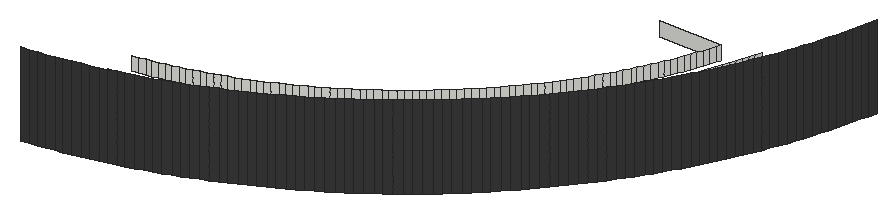
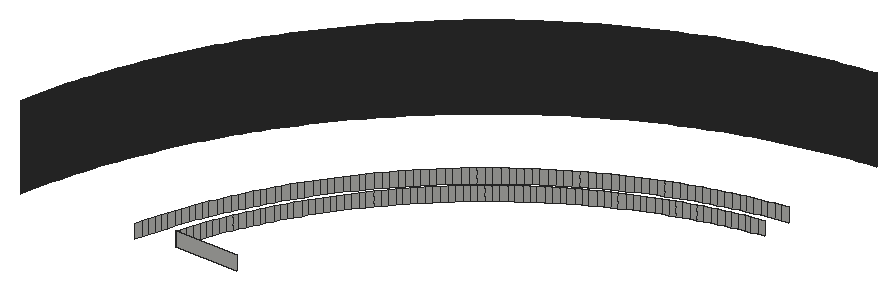
# SketchUp Ruby script. Lengths in inches.
U = 1.inch
M = Sketchup.active_model
def pt(a) = Geom::Point3d.new(a.map { |v| v * U })
def face(e, loops, mat)
  f = e.add_face(loops[0].map { |a| pt(a) })
  loops[1..].each { |l| e.add_face(l.map { |a| pt(a) }).erase! }
  f.material = f.back_material = mat if mat
  f
end
# faces: each face lists its corners as indices into pts; further lists are holes
def faces(e, pts, list, mat = nil) = list.each { |f| face(e, (f[0].is_a?(Array) ? f : [f]).map { |l| l.map { |i| pts[i] } }, mat) }
# xy, xz, yz: faces in a plane at the given z, y or x. An outline is a flat list of corners, or four numbers for a rectangle; further outlines are holes
def ring(l) = l.size == 4 ? [[l[0], l[1]], [l[2], l[1]], [l[2], l[3]], [l[0], l[3]]] : l.each_slice(2).to_a
def flat(e, list, mat, &to3) = list.each { |f| face(e, (f[0].is_a?(Array) ? f : [f]).map { |l| ring(l).map { |u, v| to3.(u, v) } }, mat) }
def xy(e, z, list, mat = nil) = flat(e, list, mat) { |x, y| [x, y, z] }
def xz(e, y, list, mat = nil) = flat(e, list, mat) { |x, z| [x, y, z] }
def yz(e, x, list, mat = nil) = flat(e, list, mat) { |y, z| [x, y, z] }
def lines(e, pts, list) = list.each { |a, b| e.add_line(pt(pts[a]), pt(pts[b])) }
# prism: a flat outline (further loops are holes) pulled along v
def prism(e, loops, v, mat = nil)
  f = face(e, loops, mat); d = Geom::Vector3d.new(v.map { |x| x * U })
  f.pushpull(f.normal.samedirection?(d) ? d.length : -d.length)
end
def box(e, o, s, mat = nil) = prism(e, [[o, [o[0] + s[0], o[1], o[2]], [o[0] + s[0], o[1] + s[1], o[2]], [o[0], o[1] + s[1], o[2]]]], [0, 0, s[2]], mat)
def at(x, y, z, deg = 0) = Geom::Transformation.translation(pt([x, y, z])) * Geom::Transformation.rotation(ORIGIN, Z_AXIS, deg.degrees)
def axes(o, x, y, z) = Geom::Transformation.new([*x, 0, *y, 0, *z, 0, *pt(o).to_a, 1])
def part(name) = M.definitions.add(name)
# library, detail: a bought-in or finely detailed component or shape, given as its bounding box
def library(name, o, s) = part(name).tap { |d| box(d.entities, o, s) }
def detail(e, o, s) = box(e.add_group.entities, o, s)
def put(e, d, t, mat = nil) = e.add_instance(d, t).tap { |i| i.material = mat if mat }
def group(e, t, mat = nil) = e.add_group.tap { |g| g.transformation = t; g.material = mat if mat }.entities
root = M.entities
M.materials.add("1496 AP 8293 CARBON COPY").color = [58, 58, 58]
xz(root,80,[[198,258,200.2,258.5]])
p = [[188.01,64.22,261],[187.74,64.18,261],[187.74,64.18,258],[188.01,64.22,258],[188.29,64.26,261],[188.29,64.26,258],
  [188.56,64.3,261],[188.56,64.3,258],[188.83,64.35,261],[188.83,64.35,258],[189.1,64.4,261],[189.1,64.4,258],
  [189.37,64.46,261],[189.37,64.46,258],[189.63,64.52,261],[189.63,64.52,258],[189.9,64.58,261],[189.9,64.58,258],
  [190.17,64.65,261],[190.17,64.65,258],[190.44,64.72,261],[190.44,64.72,258],[190.7,64.79,261],[190.7,64.79,258],
  [190.96,64.86,261],[190.96,64.86,258],[191.23,64.94,261],[191.23,64.94,258],[191.49,65.03,261],[191.49,65.03,258],
  [191.75,65.11,261],[191.75,65.11,258],[192.01,65.2,261],[192.01,65.2,258],[192.27,65.3,261],[192.27,65.3,258],
  [192.53,65.39,261],[192.53,65.39,258],[192.78,65.49,261],[192.78,65.49,258],[193.04,65.6,261],[193.04,65.6,258],
  [193.29,65.71,261],[193.29,65.71,258],[193.54,65.82,261],[193.54,65.82,258],[193.79,65.93,261],[193.79,65.93,258],
  [194.04,66.05,261],[194.04,66.05,258],[194.29,66.17,261],[194.29,66.17,258],[194.53,66.29,261],[194.53,66.29,258],
  [194.78,66.42,261],[194.78,66.42,258],[195.02,66.54,261],[195.02,66.54,258],[195.26,66.68,261],[195.26,66.68,258],
  [195.5,66.8125,261],[195.5,66.8125,258],[195.74,66.95,261],[195.74,66.95,258],[195.97,67.09,261],[195.97,67.09,258],
  [196.21,67.24,261],[196.21,67.24,258],[196.4375,67.39,261],[196.4375,67.39,258],[196.67,67.54,261],[196.67,67.54,258],
  [196.89,67.69,261],[196.89,67.69,258],[197.12,67.85,261],[197.12,67.85,258],[197.34,68.01,261],[197.34,68.01,258],
  [197.56,68.17,261],[197.56,68.17,258],[187.88,68.25,258],[187.66,68.21,258],[187.66,68.21,258.5],[187.88,68.25,258.5],
  [188.1,68.28,258],[188.1,68.28,258.5],[197.78,68.34,261],[197.78,68.34,258],[188.32,68.33,258],[188.32,68.33,258.5],
  [188.53,68.37,258],[188.53,68.37,258.5],[198,68.51,261],[198,68.51,258],[188.75,68.42,258],[188.75,68.42,258.5],
  [188.97,68.47,258],[188.97,68.47,258.5],[189.18,68.52,258],[189.18,68.52,258.5],[189.4,68.58,258],[189.4,68.58,258.5],
  [198.22,68.68,261],[198.22,68.68,258],[189.61,68.64,258],[189.61,68.64,258.5],[189.83,68.7,258],[189.83,68.7,258.5],
  [190.04,68.76,258],[190.04,68.76,258.5],[198.43,68.85,261],[198.43,68.85,258],[190.25,68.83,258],[190.25,68.83,258.5],
  [190.46,68.9,258],[190.46,68.9,258.5],[190.67,68.98,258],[190.67,68.98,258.5],[198.64,69.03,261],[198.64,69.03,258],
  [190.88,69.05,258],[190.88,69.05,258.5],[198.85,69.21,261],[198.85,69.21,258],[191.09,69.13,258],[191.09,69.13,258.5],
  [191.3,69.21,258],[191.3,69.21,258.5],[187.71,69.23,258],[187.92,69.27,258],[187.92,69.27,258.5],[187.71,69.23,258.5],
  [191.51,69.29,258],[191.51,69.29,258.5],[199.05,69.39,261],[199.05,69.39,258],[188.12,69.31,258],[188.12,69.31,258.5],
  [188.33,69.35,258],[188.33,69.35,258.5],[188.53,69.39,258],[188.53,69.39,258.5],[191.71,69.38,258],[191.71,69.38,258.5],
  [188.74,69.44,258],[188.74,69.44,258.5],[188.9375,69.49,258],[188.9375,69.49,258.5],[191.91,69.47,258],[191.91,69.47,258.5],
  [199.25,69.58,261],[199.25,69.58,258],[189.14,69.55,258],[189.14,69.55,258.5],[189.34,69.6,258],[189.34,69.6,258.5],
  [192.12,69.5625,258],[192.12,69.5625,258.5],[189.54,69.66,258],[189.54,69.66,258.5],[192.32,69.66,258],[192.32,69.66,258.5],
  [199.46,69.77,261],[199.46,69.77,258],[189.74,69.72,258],[189.74,69.72,258.5],[189.94,69.78,258],[189.94,69.78,258.5],
  [192.52,69.75,258],[192.52,69.75,258.5],[190.14,69.85,258],[190.14,69.85,258.5],[190.34,69.92,258],[190.34,69.92,258.5],
  [192.72,69.85,258],[192.72,69.85,258.5],[199.65,69.96,261],[199.65,69.96,258],[190.54,69.99,258],[190.54,69.99,258.5],
  [192.92,69.96,258],[192.92,69.96,258.5],[190.73,70.0625,258],[190.73,70.0625,258.5],[193.11,70.06,258],[193.11,70.06,258.5],
  [199.85,70.15,261],[199.85,70.15,258],[190.93,70.14,258],[190.93,70.14,258.5],[191.12,70.22,258],[191.12,70.22,258.5],
  [193.31,70.17,258],[193.31,70.17,258.5],[191.32,70.3,258],[191.32,70.3,258.5],[193.5,70.28,258],[193.5,70.28,258.5],
  [200.04,70.35,261],[200.04,70.35,258],[191.51,70.38,258],[191.51,70.38,258.5],[193.69,70.39,258],[193.69,70.39,258.5],
  [200.23,70.54,261],[200.23,70.54,258],[191.7,70.47,258],[191.7,70.47,258.5],[193.88,70.51,258],[193.88,70.51,258.5],
  [191.89,70.56,258],[191.89,70.56,258.5],[194.07,70.62,258],[194.07,70.62,258.5],[200.42,70.75,261],[200.42,70.75,258],
  [192.08,70.65,258],[192.08,70.65,258.5],[194.26,70.74,258],[194.26,70.74,258.5],[192.26,70.74,258],[192.26,70.74,258.5],
  [192.45,70.84,258],[192.45,70.84,258.5],[194.44,70.87,258],[194.44,70.87,258.5],[200.61,70.95,261],[200.61,70.95,258],
  [192.63,70.9375,258],[192.63,70.9375,258.5],[192.82,71.04,258],[192.82,71.04,258.5],[194.63,70.99,258],[194.63,70.99,258.5],
  [200.79,71.15,261],[200.79,71.15,258],[193,71.14,258],[193,71.14,258.5],[194.8125,71.12,258],[194.8125,71.12,258.5],
  [193.18,71.25,258],[193.18,71.25,258.5],[194.99,71.25,258],[194.99,71.25,258.5],[193.36,71.36,258],[193.36,71.36,258.5],
  [195.17,71.38,258],[195.17,71.38,258.5],[200.97,71.36,261],[200.97,71.36,258],[193.54,71.47,258],[193.54,71.47,258.5],
  [195.35,71.51,258],[195.35,71.51,258.5],[201.15,71.57,261],[201.15,71.57,258],[193.71,71.58,258],[193.71,71.58,258.5],
  [195.52,71.65,258],[195.52,71.65,258.5],[193.89,71.7,258],[193.89,71.7,258.5],[195.7,71.79,258],[195.7,71.79,258.5],
  [201.32,71.78,261],[201.32,71.78,258],[194.0625,71.8125,258],[194.0625,71.8125,258.5],[194.23,71.93,258],[194.23,71.93,258.5],
  [195.87,71.93,258],[195.87,71.93,258.5],[201.49,72,261],[201.49,72,258],[194.4,72.06,258],[194.4,72.06,258.5],
  [196.04,72.07,258],[196.04,72.07,258.5],[201.66,72.22,261],[201.66,72.22,258],[194.57,72.18,258],[194.57,72.18,258.5],
  [196.21,72.22,258],[196.21,72.22,258.5],[194.74,72.31,258],[194.74,72.31,258.5],[196.375,72.37,258],[196.375,72.37,258.5],
  [201.83,72.44,261],[201.83,72.44,258],[194.91,72.44,258],[194.91,72.44,258.5],[195.07,72.57,258],[195.07,72.57,258.5],
  [196.54,72.52,258],[196.54,72.52,258.5],[201.99,72.66,261],[201.99,72.66,258],[196.7,72.67,258],[196.7,72.67,258.5],
  [195.23,72.7,258],[195.23,72.7,258.5],[195.39,72.83,258],[195.39,72.83,258.5],[196.86,72.82,258],[196.86,72.82,258.5],
  [202.15,72.88,261],[202.15,72.88,258],[195.55,72.97,258],[195.55,72.97,258.5],[197.02,72.98,258],[197.02,72.98,258.5],
  [202.31,73.11,261],[202.31,73.11,258],[195.71,73.11,258],[195.71,73.11,258.5],[197.18,73.14,258],[197.18,73.14,258.5],
  [195.86,73.25,258],[195.86,73.25,258.5],[197.33,73.3,258],[197.33,73.3,258.5],[202.46,73.33,261],[202.46,73.33,258],
  [196.01,73.39,258],[196.01,73.39,258.5],[197.48,73.46,258],[197.48,73.46,258.5],[202.61,73.5625,261],[202.61,73.5625,258],
  [196.16,73.54,258],[196.16,73.54,258.5],[196.3125,73.6875,258],[196.3125,73.6875,258.5],[197.63,73.625,258],[197.63,73.625,258.5],
  [197.78,73.79,258],[197.78,73.79,258.5],[202.76,73.79,261],[202.76,73.79,258],[196.46,73.84,258],[196.46,73.84,258.5],
  [196.61,73.99,258],[196.61,73.99,258.5],[197.93,73.96,258],[197.93,73.96,258.5],[202.91,74.03,261],[202.91,74.03,258],
  [196.75,74.14,258],[196.75,74.14,258.5],[198.07,74.13,258],[198.07,74.13,258.5],[203.05,74.26,261],[203.05,74.26,258],
  [196.89,74.29,258],[196.89,74.29,258.5],[198.21,74.3,258],[198.21,74.3,258.5],[197.03,74.45,258],[197.03,74.45,258.5],
  [198.35,74.48,258],[198.35,74.48,258.5],[203.1875,74.5,261],[203.1875,74.5,258],[197.17,74.61,258],[197.17,74.61,258.5],
  [198.49,74.65,258],[198.49,74.65,258.5],[203.32,74.74,261],[203.32,74.74,258],[197.3,74.77,258],[197.3,74.77,258.5],
  [198.62,74.83,258],[198.62,74.83,258.5],[203.46,74.98,261],[203.46,74.98,258],[197.43,74.93,258],[197.43,74.93,258.5],
  [198.75,75.01,258],[198.75,75.01,258.5],[197.56,75.09,258],[197.56,75.09,258.5],[198.88,75.1875,258],[198.88,75.1875,258.5],
  [203.58,75.22,261],[203.58,75.22,258],[197.69,75.26,258],[197.69,75.26,258.5],[199.01,75.37,258],[199.01,75.37,258.5],
  [203.71,75.47,261],[203.71,75.47,258],[197.82,75.43,258],[197.82,75.43,258.5],[197.94,75.6,258],[197.94,75.6,258.5],
  [199.13,75.56,258],[199.13,75.56,258.5],[203.83,75.71,261],[203.83,75.71,258],[198.07,75.77,258],[198.07,75.77,258.5],
  [199.26,75.74,258],[199.26,75.74,258.5],[199.38,75.93,258],[199.38,75.93,258.5],[203.95,75.96,261],[203.95,75.96,258],
  [198.1875,75.9375,258],[198.1875,75.9375,258.5],[198.3,76.11,258],[198.3,76.11,258.5],[199.49,76.12,258],[199.49,76.12,258.5],
  [204.07,76.21,261],[204.07,76.21,258],[198.42,76.29,258],[198.42,76.29,258.5],[199.61,76.31,258],[199.61,76.31,258.5],
  [204.18,76.46,261],[204.18,76.46,258],[198.53,76.46,258],[198.53,76.46,258.5],[199.72,76.5,258],[199.72,76.5,258.5],
  [198.64,76.64,258],[198.64,76.64,258.5],[199.83,76.69,258],[199.83,76.69,258.5],[204.29,76.71,261],[204.29,76.71,258],
  [198.75,76.82,258],[198.75,76.82,258.5],[199.94,76.89,258],[199.94,76.89,258.5],[204.4,76.96,261],[204.4,76.96,258],
  [198.86,77,258],[198.86,77,258.5],[200.04,77.08,258],[200.04,77.08,258.5],[198.96,77.18,258],[198.96,77.18,258.5],
  [204.51,77.22,261],[204.51,77.22,258],[200.15,77.28,258],[200.15,77.28,258.5],[199.0625,77.37,258],[199.0625,77.37,258.5],
  [204.61,77.47,261],[204.61,77.47,258],[200.25,77.48,258],[200.25,77.48,258.5],[199.16,77.55,258],[199.16,77.55,258.5],
  [200.34,77.68,258],[200.34,77.68,258.5],[204.7,77.73,261],[204.7,77.73,258],[199.26,77.74,258],[199.26,77.74,258.5],
  [199.35,77.92,258],[199.35,77.92,258.5],[200.4375,77.88,258],[200.4375,77.88,258.5],[204.8,77.99,261],[204.8,77.99,258],
  [199.44,78.11,258],[199.44,78.11,258.5],[200.53,78.09,258],[200.53,78.09,258.5],[204.89,78.25,261],[204.89,78.25,258],
  [199.53,78.3,258],[199.53,78.3,258.5],[200.62,78.29,258],[200.62,78.29,258.5],[204.97,78.51,261],[204.97,78.51,258],
  [199.62,78.49,258],[199.62,78.49,258.5],[200.71,78.49,258],[200.71,78.49,258.5],[199.7,78.68,258],[199.7,78.68,258.5],
  [200.79,78.7,258],[200.79,78.7,258.5],[205.06,78.77,261],[205.06,78.77,258],[199.78,78.88,258],[199.78,78.88,258.5],
  [200.87,78.91,258],[200.87,78.91,258.5],[205.14,79.04,261],[205.14,79.04,258],[199.86,79.07,258],[199.86,79.07,258.5],
  [200.95,79.12,258],[200.95,79.12,258.5],[205.21,79.3,261],[205.21,79.3,258],[199.9375,79.27,258],[199.9375,79.27,258.5],
  [201.02,79.33,258],[201.02,79.33,258.5],[200.01,79.46,258],[200.01,79.46,258.5],[201.1,79.54,258],[201.1,79.54,258.5],
  [205.28,79.56,261],[205.28,79.56,258],[200.08,79.66,258],[200.08,79.66,258.5],[201.17,79.75,258],[201.17,79.75,258.5],
  [205.35,79.83,261],[205.35,79.83,258],[200.15,79.86,258],[200.15,79.86,258.5],[201.24,79.96,258],[201.24,79.96,258.5],
  [205.42,80.1,261],[205.42,80.1,258],[200.2,80,258],[200.2,80,258.5],[201.3,80.17,258],[201.3,80.17,258.5],
  [205.48,80.37,261],[205.48,80.37,258],[201.36,80.39,258],[201.36,80.39,258.5]]
faces(root,p,[[0,1,2,3],[4,0,3,5],[6,4,5,7],[8,6,7,9],[10,8,9,11],[12,10,11,13],[14,12,13,15],[16,14,15,17],
  [18,16,17,19],[20,18,19,21],[22,20,21,23],[24,22,23,25],[26,24,25,27],[28,26,27,29],[30,28,29,31],[32,30,31,33],
  [34,32,33,35],[36,34,35,37],[38,36,37,39],[40,38,39,41],[42,40,41,43],[44,42,43,45],[46,44,45,47],[48,46,47,49],
  [50,48,49,51],[52,50,51,53],[54,52,53,55],[56,54,55,57],[58,56,57,59],[60,58,59,61],[62,60,61,63],[64,62,63,65],
  [66,64,65,67],[68,66,67,69],[70,68,69,71],[72,70,71,73],[74,72,73,75],[76,74,75,77],[78,76,77,79],[86,78,79,87],
  [92,86,87,93],[102,92,93,103],[110,102,103,111],[118,110,111,119],[122,118,119,123],[134,122,123,135],[150,134,135,151],[162,150,151,163],
  [176,162,163,177],[186,176,177,187],[198,186,187,199],[204,198,199,205],[214,204,205,215],[226,214,215,227],[234,226,227,235],[248,234,235,249],
  [254,248,249,255],[264,254,255,265],[272,264,265,273],[278,272,273,279],[288,278,279,289],[296,288,289,297],[306,296,297,307],[312,306,307,313],
  [322,312,313,323],[328,322,323,329],[338,328,329,339],[346,338,339,347],[352,346,347,353],[362,352,353,363],[368,362,363,369],[374,368,369,375],
  [384,374,375,385],[390,384,385,391],[398,390,391,399],[406,398,399,407],[414,406,407,415],[420,414,415,421],[430,420,421,431],[436,430,431,437],
  [444,436,437,445],[450,444,445,451],[458,450,451,459],[466,458,459,467],[472,466,467,473],[478,472,473,479],[488,478,479,489],[494,488,489,495],
  [500,494,495,501],[510,500,501,511],[516,510,511,517],[522,516,517,523],[528,522,523,529]],"1496 AP 8293 CARBON COPY")
faces(root,p,[[80,81,82,83],[84,80,83,85],[88,84,85,89],[90,88,89,91],[94,90,91,95],[96,94,95,97],[98,96,97,99],[100,98,99,101],
  [104,100,101,105],[106,104,105,107],[108,106,107,109],[112,108,109,113],[114,112,113,115],[116,114,115,117],[120,116,117,121],[124,120,121,125],
  [126,124,125,127],[128,129,130,131],[132,126,127,133],[129,136,137,130],[136,138,139,137],[138,140,141,139],[142,132,133,143],[140,144,145,141],
  [144,146,147,145],[148,142,143,149],[146,152,153,147],[152,154,155,153],[156,148,149,157],[154,158,159,155],[160,156,157,161],[158,164,165,159],
  [164,166,167,165],[168,160,161,169],[166,170,171,167],[170,172,173,171],[174,168,169,175],[172,178,179,173],[180,174,175,181],[178,182,183,179],
  [184,180,181,185],[182,188,189,183],[188,190,191,189],[192,184,185,193],[190,194,195,191],[196,192,193,197],[194,200,201,195],[202,196,197,203],
  [200,206,207,201],[208,202,203,209],[206,210,211,207],[212,208,209,213],[210,216,217,211],[218,212,213,219],[216,220,221,217],[220,222,223,221],
  [224,218,219,225],[222,228,229,223],[228,230,231,229],[232,224,225,233],[230,236,237,231],[238,232,233,239],[236,240,241,237],[242,238,239,243],
  [240,244,245,241],[246,242,243,247],[244,250,251,245],[252,246,247,253],[250,256,257,251],[258,252,253,259],[256,260,261,257],[262,258,259,263],
  [260,266,267,261],[266,268,269,267],[270,262,263,271],[268,274,275,269],[276,270,271,277],[274,280,281,275],[282,276,277,283],[280,284,285,281],
  [286,282,283,287],[284,290,291,285],[290,292,293,291],[294,286,287,295],[298,294,295,299],[292,300,301,293],[300,302,303,301],[304,298,299,305],
  [302,308,309,303],[310,304,305,311],[308,314,315,309],[316,310,311,317],[314,318,319,315],[320,316,317,321],[318,324,325,319],[326,320,321,327],
  [324,330,331,325],[330,332,333,331],[334,326,327,335],[336,334,335,337],[332,340,341,333],[340,342,343,341],[344,336,337,345],[342,348,349,343],
  [350,344,345,351],[348,354,355,349],[356,350,351,357],[354,358,359,355],[360,356,357,361],[358,364,365,359],[366,360,361,367],[364,370,371,365],
  [372,366,367,373],[370,376,377,371],[378,372,373,379],[376,380,381,377],[382,378,379,383],[380,386,387,381],[388,382,383,389],[386,392,393,387],
  [392,394,395,393],[396,388,389,397],[394,400,401,395],[402,396,397,403],[404,402,403,405],[400,408,409,401],[408,410,411,409],[412,404,405,413],
  [410,416,417,411],[418,412,413,419],[416,422,423,417],[424,418,419,425],[422,426,427,423],[428,424,425,429],[426,432,433,427],[434,428,429,435],
  [432,438,439,433],[440,434,435,441],[438,442,443,439],[446,440,441,447],[442,448,449,443],[452,446,447,453],[448,454,455,449],[456,452,453,457],
  [454,460,461,455],[460,462,463,461],[464,456,457,465],[462,468,469,463],[470,464,465,471],[468,474,475,469],[476,470,471,477],[474,480,481,475],
  [482,476,477,483],[480,484,485,481],[486,482,483,487],[484,490,491,485],[492,486,487,493],[490,496,497,491],[498,492,493,499],[496,502,503,497],
  [504,498,499,505],[502,506,507,503],[508,504,505,509],[506,512,513,507],[514,508,509,515],[512,518,519,513],[520,514,515,521],[518,524,525,519],
  [526,520,521,527],[530,526,527,531]])
